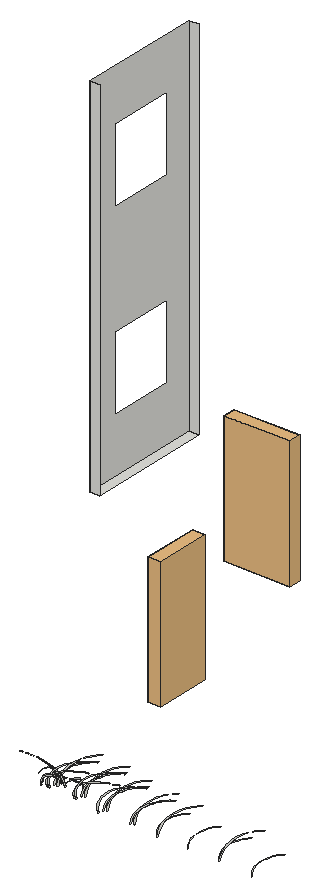
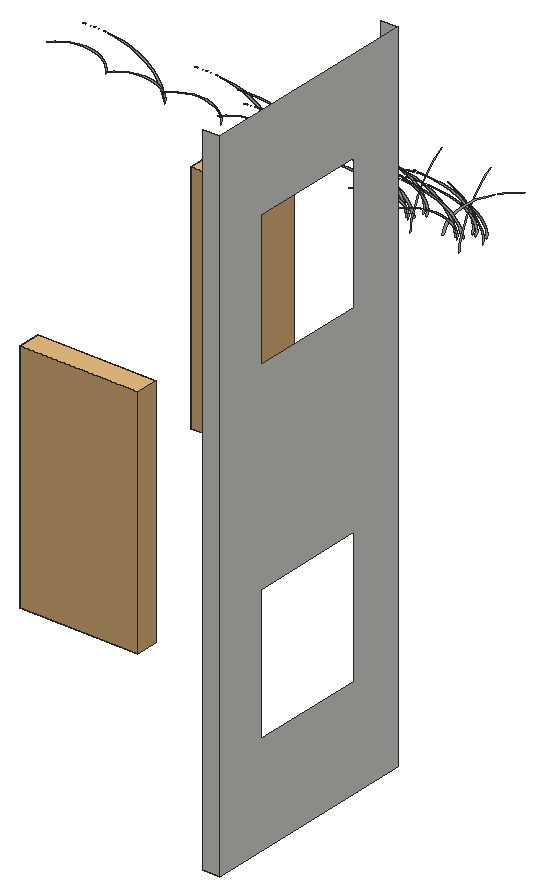
# SketchUp Ruby script. Lengths in inches.
U = 1.inch
M = Sketchup.active_model
def pt(a) = Geom::Point3d.new(a.map { |v| v * U })
def face(e, loops, mat)
  f = e.add_face(loops[0].map { |a| pt(a) })
  loops[1..].each { |l| e.add_face(l.map { |a| pt(a) }).erase! }
  f.material = f.back_material = mat if mat
  f
end
# faces: each face lists its corners as indices into pts; further lists are holes
def faces(e, pts, list, mat = nil) = list.each { |f| face(e, (f[0].is_a?(Array) ? f : [f]).map { |l| l.map { |i| pts[i] } }, mat) }
# xy, xz, yz: faces in a plane at the given z, y or x. An outline is a flat list of corners, or four numbers for a rectangle; further outlines are holes
def ring(l) = l.size == 4 ? [[l[0], l[1]], [l[2], l[1]], [l[2], l[3]], [l[0], l[3]]] : l.each_slice(2).to_a
def flat(e, list, mat, &to3) = list.each { |f| face(e, (f[0].is_a?(Array) ? f : [f]).map { |l| ring(l).map { |u, v| to3.(u, v) } }, mat) }
def xy(e, z, list, mat = nil) = flat(e, list, mat) { |x, y| [x, y, z] }
def xz(e, y, list, mat = nil) = flat(e, list, mat) { |x, z| [x, y, z] }
def yz(e, x, list, mat = nil) = flat(e, list, mat) { |y, z| [x, y, z] }
def lines(e, pts, list) = list.each { |a, b| e.add_line(pt(pts[a]), pt(pts[b])) }
# prism: a flat outline (further loops are holes) pulled along v
def prism(e, loops, v, mat = nil)
  f = face(e, loops, mat); d = Geom::Vector3d.new(v.map { |x| x * U })
  f.pushpull(f.normal.samedirection?(d) ? d.length : -d.length)
end
def box(e, o, s, mat = nil) = prism(e, [[o, [o[0] + s[0], o[1], o[2]], [o[0] + s[0], o[1] + s[1], o[2]], [o[0], o[1] + s[1], o[2]]]], [0, 0, s[2]], mat)
def at(x, y, z, deg = 0) = Geom::Transformation.translation(pt([x, y, z])) * Geom::Transformation.rotation(ORIGIN, Z_AXIS, deg.degrees)
def axes(o, x, y, z) = Geom::Transformation.new([*x, 0, *y, 0, *z, 0, *pt(o).to_a, 1])
def part(name) = M.definitions.add(name)
# library, detail: a bought-in or finely detailed component or shape, given as its bounding box
def library(name, o, s) = part(name).tap { |d| box(d.entities, o, s) }
def detail(e, o, s) = box(e.add_group.entities, o, s)
def put(e, d, t, mat = nil) = e.add_instance(d, t).tap { |i| i.material = mat if mat }
def group(e, t, mat = nil) = e.add_group.tap { |g| g.transformation = t; g.material = mat if mat }.entities
root = M.entities
c1 = library("PINTU 6 YA",[0,-0.6875,0],[35.83,8.07,80.71])
xy(root,0,[[213.74,518.03,219.74,597.83]])
xz(root,518.03,[[213.74,0,219.74,237.3]])
xz(root,597.83,[[213.74,0,219.74,237.3]])
yz(root,213.74,[[[518.03,0,597.83,237.3],[537.64,36,579.64,84],[537.64,156,579.64,204]]])
g1 = group(root,at(382.22,267.36,0))
p = [[0.99,-0.08,0],[0.44,-0.04,0],[0,0,1.49],[0.18,-0.01,2.99],[0.97,-0.08,4.45],[2.35,-0.19,5.86],
  [4.3,-0.35,7.16],[6.75,-0.55,8.33],[9.66,-0.78,9.33],[12.9375,-1.05,10.15],[16.52,-1.34,10.77],[20.31,-1.64,11.16],
  [24.21,-1.96,11.32],[28.13,-2.27,11.24],[24.28,-1.96,11.26],[20.48,-1.66,11.05],[16.8,-1.36,10.625],[13.33,-1.08,9.99],
  [10.15,-0.82,9.16],[7.34,-0.59,8.16],[4.95,-0.4,7.01],[3.05,-0.25,5.73],[1.68,-0.14,4.36],[0.87,-0.07,2.93],
  [0.64,-0.05,1.46]]
faces(g1,p,[[0,1,2,3,4,5,6,7,8,9,10,11,12,13,14,15,16,17,18,19,20,21,22,23,24]])
g2 = group(root,at(524.25,260.32,0))
p = [[11.88,11.88,11.375],[10.28,10.28,11.3],[8.71,8.71,11.03],[7.19,7.19,10.55],[5.77,5.77,9.89],[4.45,4.45,9.0625],
  [3.27,3.27,8.07],[2.25,2.25,6.9375],[1.41,1.41,5.69],[0.76,0.76,4.34],[0.33,0.33,2.93],[0.11,0.11,1.47],
  [0.11,0.11,0],[0,0,1.5],[0.14,0.14,3],[0.52,0.52,4.46],[1.13,1.13,5.85],[1.97,1.97,7.14],
  [3,3,8.3],[4.21,4.21,9.31],[5.58,5.58,10.14],[7.06,7.06,10.77],[8.625,8.625,11.19],[10.24,10.24,11.4]]
faces(g2,p,[[0,1,2,3,4,5,6,7,8,9,10,11,12,13,14,15,16,17,18,19,20,21,22,23]])
g3 = group(root,at(381.04,270.66,0))
p = [[0.69,-0.31,0],[0.31,-0.14,0],[0,0,1.24],[0.125,-0.06,2.49],[0.68,-0.3,3.72],[1.65,-0.73,4.89],
  [3.01,-1.34,5.98],[4.73,-2.11,6.95],[6.76,-3.01,7.8],[9.06,-4.04,8.48],[11.5625,-5.15,8.99],[14.21,-6.33,9.32],
  [16.94,-7.55,9.46],[19.6875,-8.77,9.39],[17,-7.58,9.4],[14.33,-6.39,9.23],[11.76,-5.24,8.875],[9.33,-4.16,8.35],
  [7.1,-3.17,7.65],[5.14,-2.29,6.82],[3.47,-1.55,5.86],[2.14,-0.95,4.79],[1.18,-0.52,3.64],[0.61,-0.27,2.45],
  [0.45,-0.2,1.22]]
faces(g3,p,[[0,1,2,3,4,5,6,7,8,9,10,11,12,13,14,15,16,17,18,19,20,21,22,23,24]])
g4 = group(root,at(401.41,278.16,0))
p = [[6.07,-19.87,14.56],[6.99,-22.87,14.94],[6.1,-19.96,14.48],[5.25,-17.16,13.83],[4.43,-14.49,13.02],[3.66,-11.97,12.04],
  [2.95,-9.65,10.91],[2.31,-7.54,9.64],[1.73,-5.67,8.25],[1.24,-4.06,6.75],[0.83,-2.72,5.15],[0.51,-1.68,3.49],
  [0.29,-0.94,1.76],[0.16,-0.52,0],[0,0,0],[0.11,-0.35,1.8],[0.32,-1.04,3.57],[0.63,-2.07,5.28],
  [1.04,-3.41,6.91],[1.55,-5.05,8.44],[2.13,-6.98,9.85],[2.8,-9.16,11.13],[3.54,-11.58,12.25],[4.34,-14.1875,13.2],
  [5.1875,-16.96,13.97]]
faces(g4,p,[[0,1,2,3,4,5,6,7,8,9,10,11,12,13,14,15,16,17,18,19,20,21,22,23,24]])
g5 = group(root,at(501.7,262.26,0))
p = [[19.18,7.98,20.75],[22.08,9.1875,21.3],[19.27,8.02,20.63],[16.57,6.9,19.72],[13.98,5.82,18.55],[11.56,4.8125,17.16],
  [9.32,3.88,15.55],[7.28,3.03,13.74],[5.47,2.28,11.76],[3.92,1.63,9.62],[2.63,1.09,7.35],[1.625,0.68,4.97],
  [0.91,0.38,2.51],[0.5,0.21,0],[0,0,0],[0.34,0.14,2.57],[1.01,0.42,5.09],[1.99,0.83,7.53],
  [3.29,1.37,9.85],[4.88,2.03,12.03],[6.74,2.81,14.04],[8.85,3.68,15.86],[11.18,4.65,17.46],[13.7,5.7,18.82],
  [16.375,6.82,19.92]]
faces(g5,p,[[0,1,2,3,4,5,6,7,8,9,10,11,12,13,14,15,16,17,18,19,20,21,22,23,24]])
g6 = group(root,at(461.5625,262.28,0))
p = [[19.18,7.98,20.75],[22.08,9.1875,21.3],[19.27,8.02,20.63],[16.57,6.9,19.72],[13.98,5.82,18.55],[11.56,4.8125,17.16],
  [9.32,3.88,15.55],[7.28,3.03,13.74],[5.47,2.28,11.76],[3.92,1.63,9.62],[2.63,1.09,7.35],[1.625,0.68,4.97],
  [0.91,0.38,2.51],[0.5,0.21,0],[0,0,0],[0.34,0.14,2.57],[1.01,0.42,5.09],[1.99,0.83,7.53],
  [3.29,1.37,9.85],[4.88,2.03,12.03],[6.74,2.81,14.04],[8.85,3.68,15.86],[11.18,4.65,17.46],[13.7,5.7,18.82],
  [16.375,6.82,19.92]]
faces(g6,p,[[0,1,2,3,4,5,6,7,8,9,10,11,12,13,14,15,16,17,18,19,20,21,22,23,24]])
g7 = group(root,at(383.55,278.58,0))
p = [[6.07,-19.87,14.56],[6.99,-22.87,14.94],[6.1,-19.96,14.48],[5.25,-17.16,13.83],[4.43,-14.49,13.02],[3.66,-11.97,12.04],
  [2.95,-9.65,10.91],[2.31,-7.54,9.64],[1.73,-5.67,8.25],[1.24,-4.06,6.75],[0.83,-2.72,5.15],[0.51,-1.68,3.49],
  [0.29,-0.94,1.76],[0.16,-0.52,0],[0,0,0],[0.11,-0.35,1.8],[0.32,-1.04,3.57],[0.63,-2.07,5.28],
  [1.04,-3.41,6.91],[1.55,-5.05,8.44],[2.13,-6.98,9.85],[2.8,-9.16,11.13],[3.54,-11.58,12.25],[4.34,-14.1875,13.2],
  [5.1875,-16.96,13.97]]
faces(g7,p,[[0,1,2,3,4,5,6,7,8,9,10,11,12,13,14,15,16,17,18,19,20,21,22,23,24]])
g8 = group(root,at(422.28,262.83,0))
p = [[0.85,0.36,0],[0.38,0.16,0],[0,0,2.37],[0.15,0.0625,4.75],[0.84,0.35,7.08],[2.03,0.85,9.32],
  [3.71,1.54,11.39],[5.83,2.42,13.25],[8.33,3.47,14.85],[11.16,4.65,16.15],[14.25,5.93,17.13],[17.52,7.29,17.75],
  [20.89,8.69,18.01],[24.27,10.1,17.89],[20.95,8.72,17.91],[17.67,7.35,17.58],[14.49,6.03,16.9],[11.5,4.79,15.89],
  [8.76,3.65,14.58],[6.33,2.63,12.99],[4.27,1.78,11.15],[2.63,1.1,9.125],[1.45,0.6,6.94],[0.75,0.3125,4.66],
  [0.55,0.23,2.33]]
faces(g8,p,[[0,1,2,3,4,5,6,7,8,9,10,11,12,13,14,15,16,17,18,19,20,21,22,23,24]])
g9 = group(root,at(393.8,273.17,0))
p = [[-19.18,-7.98,16.73],[-22.08,-9.1875,17.17],[-19.27,-8.02,16.64],[-16.57,-6.9,15.9],[-13.98,-5.82,14.96],[-11.56,-4.8125,13.84],
  [-9.32,-3.88,12.54],[-7.28,-3.03,11.08],[-5.47,-2.28,9.48],[-3.92,-1.63,7.76],[-2.63,-1.09,5.92],[-1.625,-0.68,4.01],
  [-0.91,-0.38,2.02],[-0.5,-0.21,0],[0,0,0],[-0.34,-0.14,2.07],[-1.01,-0.42,4.1],[-1.99,-0.83,6.07],
  [-3.29,-1.37,7.94],[-4.88,-2.03,9.7],[-6.74,-2.81,11.33],[-8.85,-3.68,12.79],[-11.18,-4.65,14.08],[-13.7,-5.7,15.17],
  [-16.375,-6.82,16.0625]]
faces(g9,p,[[0,1,2,3,4,5,6,7,8,9,10,11,12,13,14,15,16,17,18,19,20,21,22,23,24]])
g10 = group(root,at(481.2,262.65,0))
p = [[11.88,11.88,11.375],[10.28,10.28,11.3],[8.71,8.71,11.03],[7.19,7.19,10.55],[5.77,5.77,9.89],[4.45,4.45,9.0625],
  [3.27,3.27,8.07],[2.25,2.25,6.9375],[1.41,1.41,5.69],[0.76,0.76,4.34],[0.33,0.33,2.93],[0.11,0.11,1.47],
  [0.11,0.11,0],[0,0,1.5],[0.14,0.14,3],[0.52,0.52,4.46],[1.13,1.13,5.85],[1.97,1.97,7.14],
  [3,3,8.3],[4.21,4.21,9.31],[5.58,5.58,10.14],[7.06,7.06,10.77],[8.625,8.625,11.19],[10.24,10.24,11.4]]
faces(g10,p,[[0,1,2,3,4,5,6,7,8,9,10,11,12,13,14,15,16,17,18,19,20,21,22,23]])
g11 = group(root,at(442.47,264.1875,0))
p = [[19.18,7.98,16.73],[22.08,9.1875,17.17],[19.27,8.02,16.64],[16.57,6.9,15.9],[13.98,5.82,14.96],[11.56,4.8125,13.84],
  [9.32,3.88,12.54],[7.28,3.03,11.08],[5.47,2.28,9.48],[3.92,1.63,7.76],[2.63,1.09,5.92],[1.625,0.68,4.01],
  [0.91,0.38,2.02],[0.5,0.21,0],[0,0,0],[0.34,0.14,2.07],[1.01,0.42,4.1],[1.99,0.83,6.07],
  [3.29,1.37,7.94],[4.88,2.03,9.7],[6.74,2.81,11.33],[8.85,3.68,12.79],[11.18,4.65,14.08],[13.7,5.7,15.17],
  [16.375,6.82,16.0625]]
faces(g11,p,[[0,1,2,3,4,5,6,7,8,9,10,11,12,13,14,15,16,17,18,19,20,21,22,23,24]])
g12 = group(root,at(500.68,263.38,0))
p = [[11.88,11.88,11.375],[10.28,10.28,11.3],[8.71,8.71,11.03],[7.19,7.19,10.55],[5.77,5.77,9.89],[4.45,4.45,9.0625],
  [3.27,3.27,8.07],[2.25,2.25,6.9375],[1.41,1.41,5.69],[0.76,0.76,4.34],[0.33,0.33,2.93],[0.11,0.11,1.47],
  [0.11,0.11,0],[0,0,1.5],[0.14,0.14,3],[0.52,0.52,4.46],[1.13,1.13,5.85],[1.97,1.97,7.14],
  [3,3,8.3],[4.21,4.21,9.31],[5.58,5.58,10.14],[7.06,7.06,10.77],[8.625,8.625,11.19],[10.24,10.24,11.4]]
faces(g12,p,[[0,1,2,3,4,5,6,7,8,9,10,11,12,13,14,15,16,17,18,19,20,21,22,23]])
g13 = group(root,at(460.54,263.4,0))
p = [[11.88,11.88,11.375],[10.28,10.28,11.3],[8.71,8.71,11.03],[7.19,7.19,10.55],[5.77,5.77,9.89],[4.45,4.45,9.0625],
  [3.27,3.27,8.07],[2.25,2.25,6.9375],[1.41,1.41,5.69],[0.76,0.76,4.34],[0.33,0.33,2.93],[0.11,0.11,1.47],
  [0.11,0.11,0],[0,0,1.5],[0.14,0.14,3],[0.52,0.52,4.46],[1.13,1.13,5.85],[1.97,1.97,7.14],
  [3,3,8.3],[4.21,4.21,9.31],[5.58,5.58,10.14],[7.06,7.06,10.77],[8.625,8.625,11.19],[10.24,10.24,11.4]]
faces(g13,p,[[0,1,2,3,4,5,6,7,8,9,10,11,12,13,14,15,16,17,18,19,20,21,22,23]])
g14 = group(root,at(444.25,264.93,0))
p = [[19.18,7.98,20.75],[22.08,9.1875,21.3],[19.27,8.02,20.63],[16.57,6.9,19.72],[13.98,5.82,18.55],[11.56,4.8125,17.16],
  [9.32,3.88,15.55],[7.28,3.03,13.74],[5.47,2.28,11.76],[3.92,1.63,9.62],[2.63,1.09,7.35],[1.625,0.68,4.97],
  [0.91,0.38,2.51],[0.5,0.21,0],[0,0,0],[0.34,0.14,2.57],[1.01,0.42,5.09],[1.99,0.83,7.53],
  [3.29,1.37,9.85],[4.88,2.03,12.03],[6.74,2.81,14.04],[8.85,3.68,15.86],[11.18,4.65,17.46],[13.7,5.7,18.82],
  [16.375,6.82,19.92]]
faces(g14,p,[[0,1,2,3,4,5,6,7,8,9,10,11,12,13,14,15,16,17,18,19,20,21,22,23,24]])
g15 = group(root,at(403.17,267.64,0))
p = [[0.91,0.18,0],[0.4,0.08,0],[0,0,1.75],[0.16,0.03,3.51],[0.89,0.17,5.24],[2.16,0.42,6.89],
  [3.94,0.76,8.42],[6.19,1.2,9.8],[8.86,1.72,10.98],[11.87,2.3,11.95],[15.16,2.94,12.67],[18.63,3.61,13.13],
  [22.21,4.31,13.32],[25.81,5.01,13.23],[22.28,4.32,13.25],[18.79,3.64,13],[15.41,2.99,12.5],[12.23,2.37,11.75],
  [9.3125,1.81,10.78],[6.73,1.31,9.6],[4.54,0.88,8.25],[2.8,0.54,6.75],[1.54,0.3,5.13],[0.8,0.16,3.44],
  [0.59,0.11,1.72]]
faces(g15,p,[[0,1,2,3,4,5,6,7,8,9,10,11,12,13,14,15,16,17,18,19,20,21,22,23,24]])
g16 = group(root,at(385.31,268.06,0))
p = [[0.91,0.18,0],[0.4,0.08,0],[0,0,1.75],[0.16,0.03,3.51],[0.89,0.17,5.24],[2.16,0.42,6.89],
  [3.94,0.76,8.42],[6.19,1.2,9.8],[8.86,1.72,10.98],[11.87,2.3,11.95],[15.16,2.94,12.67],[18.63,3.61,13.13],
  [22.21,4.31,13.32],[25.81,5.01,13.23],[22.28,4.32,13.25],[18.79,3.64,13],[15.41,2.99,12.5],[12.23,2.37,11.75],
  [9.3125,1.81,10.78],[6.73,1.31,9.6],[4.54,0.88,8.25],[2.8,0.54,6.75],[1.54,0.3,5.13],[0.8,0.16,3.44],
  [0.59,0.11,1.72]]
faces(g16,p,[[0,1,2,3,4,5,6,7,8,9,10,11,12,13,14,15,16,17,18,19,20,21,22,23,24]])
g17 = group(root,at(423.32,266.4,0))
p = [[19.18,7.98,16.73],[22.08,9.1875,17.17],[19.27,8.02,16.64],[16.57,6.9,15.9],[13.98,5.82,14.96],[11.56,4.8125,13.84],
  [9.32,3.88,12.54],[7.28,3.03,11.08],[5.47,2.28,9.48],[3.92,1.63,7.76],[2.63,1.09,5.92],[1.625,0.68,4.01],
  [0.91,0.38,2.02],[0.5,0.21,0],[0,0,0],[0.34,0.14,2.07],[1.01,0.42,4.1],[1.99,0.83,6.07],
  [3.29,1.37,7.94],[4.88,2.03,9.7],[6.74,2.81,11.33],[8.85,3.68,12.79],[11.18,4.65,14.08],[13.7,5.7,15.17],
  [16.375,6.82,16.0625]]
faces(g17,p,[[0,1,2,3,4,5,6,7,8,9,10,11,12,13,14,15,16,17,18,19,20,21,22,23,24]])
g18 = group(root,at(425.1,267.15,0))
p = [[19.18,7.98,20.75],[22.08,9.1875,21.3],[19.27,8.02,20.63],[16.57,6.9,19.72],[13.98,5.82,18.55],[11.56,4.8125,17.16],
  [9.32,3.88,15.55],[7.28,3.03,13.74],[5.47,2.28,11.76],[3.92,1.63,9.62],[2.63,1.09,7.35],[1.625,0.68,4.97],
  [0.91,0.38,2.51],[0.5,0.21,0],[0,0,0],[0.34,0.14,2.57],[1.01,0.42,5.09],[1.99,0.83,7.53],
  [3.29,1.37,9.85],[4.88,2.03,12.03],[6.74,2.81,14.04],[8.85,3.68,15.86],[11.18,4.65,17.46],[13.7,5.7,18.82],
  [16.375,6.82,19.92]]
faces(g18,p,[[0,1,2,3,4,5,6,7,8,9,10,11,12,13,14,15,16,17,18,19,20,21,22,23,24]])
g19 = group(root,at(443.23,266.06,0))
p = [[11.88,11.88,11.375],[10.28,10.28,11.3],[8.71,8.71,11.03],[7.19,7.19,10.55],[5.77,5.77,9.89],[4.45,4.45,9.0625],
  [3.27,3.27,8.07],[2.25,2.25,6.9375],[1.41,1.41,5.69],[0.76,0.76,4.34],[0.33,0.33,2.93],[0.11,0.11,1.47],
  [0.11,0.11,0],[0,0,1.5],[0.14,0.14,3],[0.52,0.52,4.46],[1.13,1.13,5.85],[1.97,1.97,7.14],
  [3,3,8.3],[4.21,4.21,9.31],[5.58,5.58,10.14],[7.06,7.06,10.77],[8.625,8.625,11.19],[10.24,10.24,11.4]]
faces(g19,p,[[0,1,2,3,4,5,6,7,8,9,10,11,12,13,14,15,16,17,18,19,20,21,22,23]])
g20 = group(root,at(404.57,267.18,0))
p = [[0.85,0.36,0],[0.38,0.16,0],[0,0,2.37],[0.15,0.0625,4.75],[0.84,0.35,7.08],[2.03,0.85,9.32],
  [3.71,1.54,11.39],[5.83,2.42,13.25],[8.33,3.47,14.85],[11.16,4.65,16.15],[14.25,5.93,17.13],[17.52,7.29,17.75],
  [20.89,8.69,18.01],[24.27,10.1,17.89],[20.95,8.72,17.91],[17.67,7.35,17.58],[14.49,6.03,16.9],[11.5,4.79,15.89],
  [8.76,3.65,14.58],[6.33,2.63,12.99],[4.27,1.78,11.15],[2.63,1.1,9.125],[1.45,0.6,6.94],[0.75,0.3125,4.66],
  [0.55,0.23,2.33]]
faces(g20,p,[[0,1,2,3,4,5,6,7,8,9,10,11,12,13,14,15,16,17,18,19,20,21,22,23,24]])
g21 = group(root,at(386.71,267.6,0))
p = [[0.85,0.36,0],[0.38,0.16,0],[0,0,2.37],[0.15,0.0625,4.75],[0.84,0.35,7.08],[2.03,0.85,9.32],
  [3.71,1.54,11.39],[5.83,2.42,13.25],[8.33,3.47,14.85],[11.16,4.65,16.15],[14.25,5.93,17.13],[17.52,7.29,17.75],
  [20.89,8.69,18.01],[24.27,10.1,17.89],[20.95,8.72,17.91],[17.67,7.35,17.58],[14.49,6.03,16.9],[11.5,4.79,15.89],
  [8.76,3.65,14.58],[6.33,2.63,12.99],[4.27,1.78,11.15],[2.63,1.1,9.125],[1.45,0.6,6.94],[0.75,0.3125,4.66],
  [0.55,0.23,2.33]]
faces(g21,p,[[0,1,2,3,4,5,6,7,8,9,10,11,12,13,14,15,16,17,18,19,20,21,22,23,24]])
g22 = group(root,at(424.08,268.27,0))
p = [[11.88,11.88,11.375],[10.28,10.28,11.3],[8.71,8.71,11.03],[7.19,7.19,10.55],[5.77,5.77,9.89],[4.45,4.45,9.0625],
  [3.27,3.27,8.07],[2.25,2.25,6.9375],[1.41,1.41,5.69],[0.76,0.76,4.34],[0.33,0.33,2.93],[0.11,0.11,1.47],
  [0.11,0.11,0],[0,0,1.5],[0.14,0.14,3],[0.52,0.52,4.46],[1.13,1.13,5.85],[1.97,1.97,7.14],
  [3,3,8.3],[4.21,4.21,9.31],[5.58,5.58,10.14],[7.06,7.06,10.77],[8.625,8.625,11.19],[10.24,10.24,11.4]]
faces(g22,p,[[0,1,2,3,4,5,6,7,8,9,10,11,12,13,14,15,16,17,18,19,20,21,22,23]])
g23 = group(root,at(405.61,270.75,0))
p = [[19.18,7.98,16.73],[22.08,9.1875,17.17],[19.27,8.02,16.64],[16.57,6.9,15.9],[13.98,5.82,14.96],[11.56,4.8125,13.84],
  [9.32,3.88,12.54],[7.28,3.03,11.08],[5.47,2.28,9.48],[3.92,1.63,7.76],[2.63,1.09,5.92],[1.625,0.68,4.01],
  [0.91,0.38,2.02],[0.5,0.21,0],[0,0,0],[0.34,0.14,2.07],[1.01,0.42,4.1],[1.99,0.83,6.07],
  [3.29,1.37,7.94],[4.88,2.03,9.7],[6.74,2.81,11.33],[8.85,3.68,12.79],[11.18,4.65,14.08],[13.7,5.7,15.17],
  [16.375,6.82,16.0625]]
faces(g23,p,[[0,1,2,3,4,5,6,7,8,9,10,11,12,13,14,15,16,17,18,19,20,21,22,23,24]])
g24 = group(root,at(387.74,271.17,0))
p = [[19.18,7.98,16.73],[22.08,9.1875,17.17],[19.27,8.02,16.64],[16.57,6.9,15.9],[13.98,5.82,14.96],[11.56,4.8125,13.84],
  [9.32,3.88,12.54],[7.28,3.03,11.08],[5.47,2.28,9.48],[3.92,1.63,7.76],[2.63,1.09,5.92],[1.625,0.68,4.01],
  [0.91,0.38,2.02],[0.5,0.21,0],[0,0,0],[0.34,0.14,2.07],[1.01,0.42,4.1],[1.99,0.83,6.07],
  [3.29,1.37,7.94],[4.88,2.03,9.7],[6.74,2.81,11.33],[8.85,3.68,12.79],[11.18,4.65,14.08],[13.7,5.7,15.17],
  [16.375,6.82,16.0625]]
faces(g24,p,[[0,1,2,3,4,5,6,7,8,9,10,11,12,13,14,15,16,17,18,19,20,21,22,23,24]])
g25 = group(root,at(407.39,271.5,0))
p = [[19.18,7.98,20.75],[22.08,9.1875,21.3],[19.27,8.02,20.63],[16.57,6.9,19.72],[13.98,5.82,18.55],[11.56,4.8125,17.16],
  [9.32,3.88,15.55],[7.28,3.03,13.74],[5.47,2.28,11.76],[3.92,1.63,9.62],[2.63,1.09,7.35],[1.625,0.68,4.97],
  [0.91,0.38,2.51],[0.5,0.21,0],[0,0,0],[0.34,0.14,2.57],[1.01,0.42,5.09],[1.99,0.83,7.53],
  [3.29,1.37,9.85],[4.88,2.03,12.03],[6.74,2.81,14.04],[8.85,3.68,15.86],[11.18,4.65,17.46],[13.7,5.7,18.82],
  [16.375,6.82,19.92]]
faces(g25,p,[[0,1,2,3,4,5,6,7,8,9,10,11,12,13,14,15,16,17,18,19,20,21,22,23,24]])
g26 = group(root,at(389.53,271.91,0))
p = [[19.18,7.98,20.75],[22.08,9.1875,21.3],[19.27,8.02,20.63],[16.57,6.9,19.72],[13.98,5.82,18.55],[11.56,4.8125,17.16],
  [9.32,3.88,15.55],[7.28,3.03,13.74],[5.47,2.28,11.76],[3.92,1.63,9.62],[2.63,1.09,7.35],[1.625,0.68,4.97],
  [0.91,0.38,2.51],[0.5,0.21,0],[0,0,0],[0.34,0.14,2.57],[1.01,0.42,5.09],[1.99,0.83,7.53],
  [3.29,1.37,9.85],[4.88,2.03,12.03],[6.74,2.81,14.04],[8.85,3.68,15.86],[11.18,4.65,17.46],[13.7,5.7,18.82],
  [16.375,6.82,19.92]]
faces(g26,p,[[0,1,2,3,4,5,6,7,8,9,10,11,12,13,14,15,16,17,18,19,20,21,22,23,24]])
g27 = group(root,at(406.37,272.62,0))
p = [[11.88,11.88,11.375],[10.28,10.28,11.3],[8.71,8.71,11.03],[7.19,7.19,10.55],[5.77,5.77,9.89],[4.45,4.45,9.0625],
  [3.27,3.27,8.07],[2.25,2.25,6.9375],[1.41,1.41,5.69],[0.76,0.76,4.34],[0.33,0.33,2.93],[0.11,0.11,1.47],
  [0.11,0.11,0],[0,0,1.5],[0.14,0.14,3],[0.52,0.52,4.46],[1.13,1.13,5.85],[1.97,1.97,7.14],
  [3,3,8.3],[4.21,4.21,9.31],[5.58,5.58,10.14],[7.06,7.06,10.77],[8.625,8.625,11.19],[10.24,10.24,11.4]]
faces(g27,p,[[0,1,2,3,4,5,6,7,8,9,10,11,12,13,14,15,16,17,18,19,20,21,22,23]])
g28 = group(root,at(388.51,273.04,0))
p = [[11.88,11.88,11.375],[10.28,10.28,11.3],[8.71,8.71,11.03],[7.19,7.19,10.55],[5.77,5.77,9.89],[4.45,4.45,9.0625],
  [3.27,3.27,8.07],[2.25,2.25,6.9375],[1.41,1.41,5.69],[0.76,0.76,4.34],[0.33,0.33,2.93],[0.11,0.11,1.47],
  [0.11,0.11,0],[0,0,1.5],[0.14,0.14,3],[0.52,0.52,4.46],[1.13,1.13,5.85],[1.97,1.97,7.14],
  [3,3,8.3],[4.21,4.21,9.31],[5.58,5.58,10.14],[7.06,7.06,10.77],[8.625,8.625,11.19],[10.24,10.24,11.4]]
faces(g28,p,[[0,1,2,3,4,5,6,7,8,9,10,11,12,13,14,15,16,17,18,19,20,21,22,23]])
put(root,c1,axes([372.21,403.35,0],[0,-1,0],[1,0,0],[0,0,1.04]))
put(root,c1,axes([310.83,505.52,0],[1.18,0,0],[0,1,0],[0,0,1.04]))
